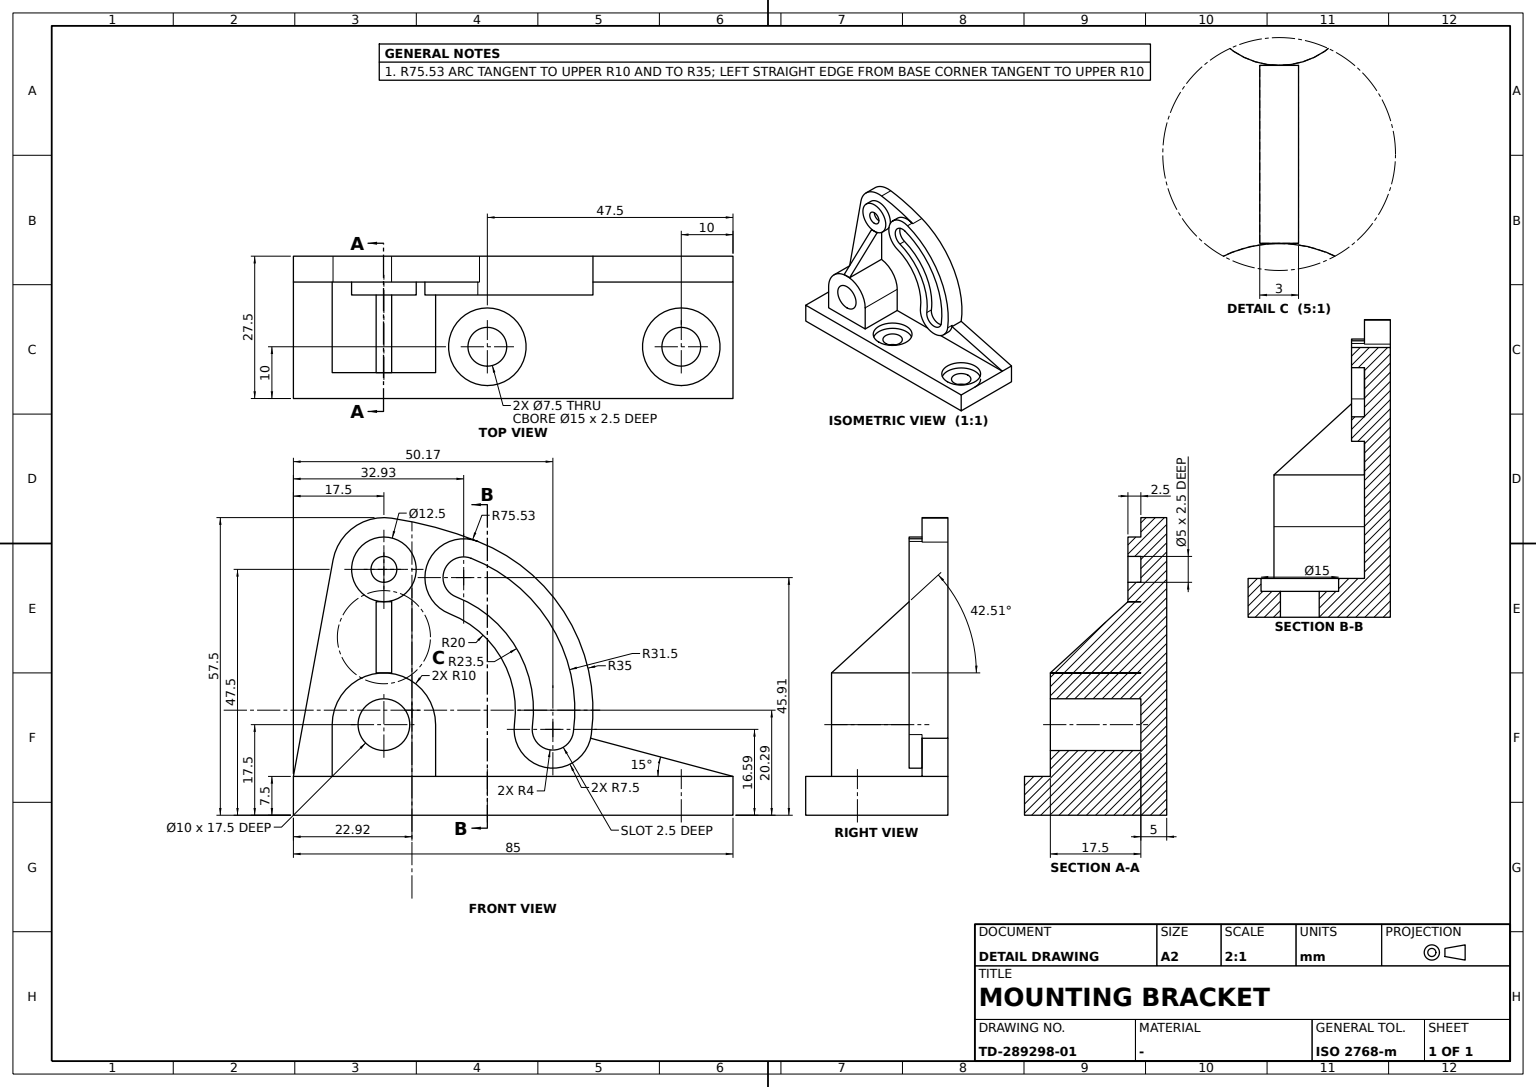
ISO-10303-21;
HEADER;
FILE_DESCRIPTION((''),'2;1');
FILE_NAME('','',(''),(''),'','','');
FILE_SCHEMA(('AUTOMOTIVE_DESIGN'));
ENDSEC;
DATA;
#1=APPLICATION_CONTEXT('');
#2=PRODUCT_CONTEXT('',#1,'mechanical');
#3=PRODUCT('','','',(#2));
#4=PRODUCT_DEFINITION_FORMATION('','',#3);
#5=PRODUCT_DEFINITION_CONTEXT('',#1,'design');
#6=PRODUCT_DEFINITION('','',#4,#5);
#7=PRODUCT_DEFINITION_SHAPE('','',#6);
#8=(LENGTH_UNIT()NAMED_UNIT(*)SI_UNIT(.MILLI.,.METRE.));
#9=(NAMED_UNIT(*)PLANE_ANGLE_UNIT()SI_UNIT($,.RADIAN.));
#10=(NAMED_UNIT(*)SI_UNIT($,.STERADIAN.)SOLID_ANGLE_UNIT());
#11=UNCERTAINTY_MEASURE_WITH_UNIT(LENGTH_MEASURE(0.005),#8,'distance_accuracy_value','');
#12=(GEOMETRIC_REPRESENTATION_CONTEXT(3)GLOBAL_UNCERTAINTY_ASSIGNED_CONTEXT((#11))GLOBAL_UNIT_ASSIGNED_CONTEXT((#8,#9,#10))REPRESENTATION_CONTEXT('',''));
#13=CARTESIAN_POINT('',(-3.75,-5.,5.));
#14=VERTEX_POINT('',#13);
#15=CARTESIAN_POINT('',(3.75,-5.,5.));
#16=DIRECTION('',(0.,0.,-1.));
#17=DIRECTION('',(-1.,0.,0.));
#18=AXIS2_PLACEMENT_3D('',#15,#16,#17);
#19=CIRCLE('',#18,7.5);
#20=EDGE_CURVE('',#14,#14,#19,.T.);
#21=ORIENTED_EDGE('',*,*,#20,.F.);
#22=EDGE_LOOP('',(#21));
#23=FACE_BOUND('',#22,.T.);
#24=CARTESIAN_POINT('',(0.,-5.,5.));
#25=VERTEX_POINT('',#24);
#26=CIRCLE('',#18,3.75);
#27=EDGE_CURVE('',#25,#25,#26,.T.);
#28=ORIENTED_EDGE('',*,*,#27,.T.);
#29=EDGE_LOOP('',(#28));
#30=FACE_BOUND('',#29,.T.);
#31=CARTESIAN_POINT('',(7.5,32.5,5.));
#32=DIRECTION('',(1.,0.,0.));
#33=AXIS2_PLACEMENT_3D('',#31,#16,#32);
#34=PLANE('',#33);
#35=ADVANCED_FACE('',(#23,#30),#34,.F.);
#36=CARTESIAN_POINT('',(13.75,42.5,0.));
#37=VERTEX_POINT('',#36);
#38=CARTESIAN_POINT('',(13.75,-42.5,0.));
#39=VERTEX_POINT('',#38);
#40=CARTESIAN_POINT('',(13.75,0.,0.));
#41=DIRECTION('',(0.,-1.,0.));
#42=VECTOR('',#41,1000.);
#43=LINE('',#40,#42);
#44=EDGE_CURVE('',#37,#39,#43,.T.);
#45=ORIENTED_EDGE('',*,*,#44,.F.);
#46=CARTESIAN_POINT('',(13.75,42.5,7.5));
#47=VERTEX_POINT('',#46);
#48=DIRECTION('',(0.,0.,1.));
#49=VECTOR('',#48,1000.);
#50=LINE('',#36,#49);
#51=EDGE_CURVE('',#37,#47,#50,.T.);
#52=ORIENTED_EDGE('',*,*,#51,.T.);
#53=CARTESIAN_POINT('',(13.75,-42.5,7.5));
#54=VERTEX_POINT('',#53);
#55=CARTESIAN_POINT('',(13.75,0.,7.5));
#56=LINE('',#55,#42);
#57=EDGE_CURVE('',#47,#54,#56,.T.);
#58=ORIENTED_EDGE('',*,*,#57,.T.);
#59=LINE('',#38,#49);
#60=EDGE_CURVE('',#39,#54,#59,.T.);
#61=ORIENTED_EDGE('',*,*,#60,.F.);
#62=EDGE_LOOP('',(#45,#52,#58,#61));
#63=FACE_BOUND('',#62,.T.);
#64=AXIS2_PLACEMENT_3D('',#36,#17,#41);
#65=PLANE('',#64);
#66=ADVANCED_FACE('',(#63),#65,.F.);
#67=CARTESIAN_POINT('',(-13.75,-34.836066,49.303279));
#68=VERTEX_POINT('',#67);
#69=CARTESIAN_POINT('',(-13.75,-42.5,7.5));
#70=VERTEX_POINT('',#69);
#71=CARTESIAN_POINT('',(-13.75,-43.830288,0.243886));
#72=DIRECTION('',(0.,-0.180327869,-0.983606557));
#73=VECTOR('',#72,1000.);
#74=LINE('',#71,#73);
#75=EDGE_CURVE('',#68,#70,#74,.T.);
#76=ORIENTED_EDGE('',*,*,#75,.T.);
#77=CARTESIAN_POINT('',(-8.75,-42.5,7.5));
#78=VERTEX_POINT('',#77);
#79=VECTOR('',#32,1000.);
#80=LINE('',#53,#79);
#81=EDGE_CURVE('',#70,#78,#80,.T.);
#82=ORIENTED_EDGE('',*,*,#81,.T.);
#83=CARTESIAN_POINT('',(-8.75,-34.836066,49.303279));
#84=VERTEX_POINT('',#83);
#85=LINE('',#83,#73);
#86=EDGE_CURVE('',#84,#78,#85,.T.);
#87=ORIENTED_EDGE('',*,*,#86,.F.);
#88=CARTESIAN_POINT('',(-11.25,-34.836066,49.303279));
#89=VECTOR('',#17,1000.);
#90=LINE('',#88,#89);
#91=EDGE_CURVE('',#68,#84,#90,.F.);
#92=ORIENTED_EDGE('',*,*,#91,.F.);
#93=EDGE_LOOP('',(#76,#82,#87,#92));
#94=FACE_BOUND('',#93,.T.);
#95=DIRECTION('',(0.,-0.983606557,0.180327869));
#96=AXIS2_PLACEMENT_3D('',#67,#95,#72);
#97=PLANE('',#96);
#98=ADVANCED_FACE('',(#94),#97,.T.);
#99=CARTESIAN_POINT('',(-13.75,-42.5,0.));
#100=VERTEX_POINT('',#99);
#101=CARTESIAN_POINT('',(0.,-42.5,0.));
#102=LINE('',#101,#89);
#103=EDGE_CURVE('',#39,#100,#102,.T.);
#104=ORIENTED_EDGE('',*,*,#103,.F.);
#105=ORIENTED_EDGE('',*,*,#60,.T.);
#106=CARTESIAN_POINT('',(0.,-42.5,7.5));
#107=LINE('',#106,#89);
#108=EDGE_CURVE('',#54,#78,#107,.T.);
#109=ORIENTED_EDGE('',*,*,#108,.T.);
#110=ORIENTED_EDGE('',*,*,#81,.F.);
#111=LINE('',#99,#49);
#112=EDGE_CURVE('',#100,#70,#111,.T.);
#113=ORIENTED_EDGE('',*,*,#112,.F.);
#114=EDGE_LOOP('',(#104,#105,#109,#110,#113));
#115=FACE_BOUND('',#114,.T.);
#116=DIRECTION('',(0.,1.,0.));
#117=AXIS2_PLACEMENT_3D('',#38,#116,#17);
#118=PLANE('',#117);
#119=ADVANCED_FACE('',(#115),#118,.F.);
#120=CARTESIAN_POINT('',(7.5,32.5,0.));
#121=VERTEX_POINT('',#120);
#122=CARTESIAN_POINT('',(3.75,32.5,0.));
#123=AXIS2_PLACEMENT_3D('',#122,#48,#32);
#124=CIRCLE('',#123,3.75);
#125=EDGE_CURVE('',#121,#121,#124,.T.);
#126=ORIENTED_EDGE('',*,*,#125,.F.);
#127=EDGE_LOOP('',(#126));
#128=FACE_BOUND('',#127,.T.);
#129=CARTESIAN_POINT('',(0.,32.5,5.));
#130=VERTEX_POINT('',#129);
#131=CARTESIAN_POINT('',(3.75,32.5,5.));
#132=AXIS2_PLACEMENT_3D('',#131,#16,#17);
#133=CIRCLE('',#132,3.75);
#134=EDGE_CURVE('',#130,#130,#133,.T.);
#135=ORIENTED_EDGE('',*,*,#134,.F.);
#136=EDGE_LOOP('',(#135));
#137=FACE_BOUND('',#136,.T.);
#138=CARTESIAN_POINT('',(3.75,32.5,7.4));
#139=AXIS2_PLACEMENT_3D('',#138,#16,#32);
#140=CYLINDRICAL_SURFACE('',#139,3.75);
#141=ADVANCED_FACE('',(#128,#137),#140,.F.);
#142=CARTESIAN_POINT('',(-8.75,-15.,17.5));
#143=VERTEX_POINT('',#142);
#144=CARTESIAN_POINT('',(-8.75,-15.,7.5));
#145=VERTEX_POINT('',#144);
#146=VECTOR('',#16,1000.);
#147=LINE('',#142,#146);
#148=EDGE_CURVE('',#143,#145,#147,.T.);
#149=ORIENTED_EDGE('',*,*,#148,.T.);
#150=CARTESIAN_POINT('',(-8.75,42.5,7.5));
#151=VERTEX_POINT('',#150);
#152=CARTESIAN_POINT('',(-8.75,0.,7.5));
#153=LINE('',#152,#42);
#154=EDGE_CURVE('',#151,#145,#153,.T.);
#155=ORIENTED_EDGE('',*,*,#154,.F.);
#156=CARTESIAN_POINT('',(-8.75,14.986884,14.871731));
#157=VERTEX_POINT('',#156);
#158=DIRECTION('',(0.,-0.965925826,0.258819045));
#159=VECTOR('',#158,1000.);
#160=LINE('',#150,#159);
#161=EDGE_CURVE('',#151,#157,#160,.T.);
#162=ORIENTED_EDGE('',*,*,#161,.T.);
#163=CARTESIAN_POINT('',(-8.75,0.24077,17.599853));
#164=VERTEX_POINT('',#163);
#165=CARTESIAN_POINT('',(-8.75,7.672397,16.589451));
#166=AXIS2_PLACEMENT_3D('',#165,#17,#48);
#167=CIRCLE('',#166,7.5);
#168=EDGE_CURVE('',#164,#157,#167,.F.);
#169=ORIENTED_EDGE('',*,*,#168,.F.);
#170=CARTESIAN_POINT('',(-8.75,-12.300381,38.923598));
#171=VERTEX_POINT('',#170);
#172=CARTESIAN_POINT('',(-8.75,-19.576903,20.29426));
#173=AXIS2_PLACEMENT_3D('',#172,#17,#48);
#174=CIRCLE('',#173,20.);
#175=EDGE_CURVE('',#164,#171,#174,.F.);
#176=ORIENTED_EDGE('',*,*,#175,.T.);
#177=CARTESIAN_POINT('',(-8.75,-6.842813,52.896043));
#178=VERTEX_POINT('',#177);
#179=CARTESIAN_POINT('',(-8.75,-9.571685,45.9096));
#180=AXIS2_PLACEMENT_3D('',#179,#17,#48);
#181=CIRCLE('',#180,7.5);
#182=EDGE_CURVE('',#178,#171,#181,.F.);
#183=ORIENTED_EDGE('',*,*,#182,.F.);
#184=CARTESIAN_POINT('',(-8.75,-23.519463,57.389793));
#185=VERTEX_POINT('',#184);
#186=CARTESIAN_POINT('',(-8.75,-34.702133,-17.308958));
#187=AXIS2_PLACEMENT_3D('',#186,#17,#48);
#188=CIRCLE('',#187,75.531156);
#189=EDGE_CURVE('',#185,#178,#188,.T.);
#190=ORIENTED_EDGE('',*,*,#189,.F.);
#191=CARTESIAN_POINT('',(-8.75,-25.,47.5));
#192=AXIS2_PLACEMENT_3D('',#191,#17,#48);
#193=CIRCLE('',#192,10.);
#194=EDGE_CURVE('',#84,#185,#193,.T.);
#195=ORIENTED_EDGE('',*,*,#194,.F.);
#196=ORIENTED_EDGE('',*,*,#86,.T.);
#197=CARTESIAN_POINT('',(-8.75,-35.,7.5));
#198=VERTEX_POINT('',#197);
#199=EDGE_CURVE('',#198,#78,#153,.T.);
#200=ORIENTED_EDGE('',*,*,#199,.F.);
#201=CARTESIAN_POINT('',(-8.75,-35.,17.5));
#202=VERTEX_POINT('',#201);
#203=LINE('',#201,#146);
#204=EDGE_CURVE('',#202,#198,#203,.T.);
#205=ORIENTED_EDGE('',*,*,#204,.F.);
#206=CARTESIAN_POINT('',(-8.75,-25.,27.5));
#207=VERTEX_POINT('',#206);
#208=CARTESIAN_POINT('',(-8.75,-25.,17.5));
#209=AXIS2_PLACEMENT_3D('',#208,#17,#48);
#210=CIRCLE('',#209,10.);
#211=EDGE_CURVE('',#202,#207,#210,.T.);
#212=ORIENTED_EDGE('',*,*,#211,.T.);
#213=CARTESIAN_POINT('',(-8.75,-26.5,27.5));
#214=VERTEX_POINT('',#213);
#215=VECTOR('',#116,1000.);
#216=LINE('',#206,#215);
#217=EDGE_CURVE('',#214,#207,#216,.T.);
#218=ORIENTED_EDGE('',*,*,#217,.F.);
#219=CARTESIAN_POINT('',(-8.75,-26.5,41.25));
#220=VERTEX_POINT('',#219);
#221=CARTESIAN_POINT('',(-8.75,-26.5,0.));
#222=LINE('',#221,#146);
#223=EDGE_CURVE('',#220,#214,#222,.T.);
#224=ORIENTED_EDGE('',*,*,#223,.F.);
#225=CARTESIAN_POINT('',(-8.75,-25.,41.25));
#226=VERTEX_POINT('',#225);
#227=LINE('',#225,#215);
#228=EDGE_CURVE('',#220,#226,#227,.T.);
#229=ORIENTED_EDGE('',*,*,#228,.T.);
#230=CIRCLE('',#192,6.25);
#231=EDGE_CURVE('',#226,#226,#230,.T.);
#232=ORIENTED_EDGE('',*,*,#231,.T.);
#233=CARTESIAN_POINT('',(-8.75,-23.5,41.25));
#234=VERTEX_POINT('',#233);
#235=EDGE_CURVE('',#226,#234,#227,.T.);
#236=ORIENTED_EDGE('',*,*,#235,.T.);
#237=CARTESIAN_POINT('',(-8.75,-23.5,27.5));
#238=VERTEX_POINT('',#237);
#239=CARTESIAN_POINT('',(-8.75,-23.5,0.));
#240=LINE('',#239,#146);
#241=EDGE_CURVE('',#234,#238,#240,.T.);
#242=ORIENTED_EDGE('',*,*,#241,.T.);
#243=EDGE_CURVE('',#207,#238,#216,.T.);
#244=ORIENTED_EDGE('',*,*,#243,.F.);
#245=EDGE_CURVE('',#207,#143,#210,.T.);
#246=ORIENTED_EDGE('',*,*,#245,.T.);
#247=EDGE_LOOP('',(#149,#155,#162,#169,#176,#183,#190,#195,#196,#200,#205,#212,#218,#224,#229,#232,#236,#242,#244,#246));
#248=FACE_BOUND('',#247,.T.);
#249=CARTESIAN_POINT('',(-8.75,0.,0.));
#250=AXIS2_PLACEMENT_3D('',#249,#17,#41);
#251=PLANE('',#250);
#252=ADVANCED_FACE('',(#248),#251,.F.);
#253=CARTESIAN_POINT('',(7.5,-5.,0.));
#254=VERTEX_POINT('',#253);
#255=CARTESIAN_POINT('',(3.75,-5.,0.));
#256=AXIS2_PLACEMENT_3D('',#255,#48,#32);
#257=CIRCLE('',#256,3.75);
#258=EDGE_CURVE('',#254,#254,#257,.T.);
#259=ORIENTED_EDGE('',*,*,#258,.F.);
#260=EDGE_LOOP('',(#259));
#261=FACE_BOUND('',#260,.T.);
#262=ORIENTED_EDGE('',*,*,#27,.F.);
#263=EDGE_LOOP('',(#262));
#264=FACE_BOUND('',#263,.T.);
#265=CARTESIAN_POINT('',(3.75,-5.,7.4));
#266=AXIS2_PLACEMENT_3D('',#265,#16,#32);
#267=CYLINDRICAL_SURFACE('',#266,3.75);
#268=ADVANCED_FACE('',(#261,#264),#267,.F.);
#269=CARTESIAN_POINT('',(-6.25,-26.5,41.25));
#270=VERTEX_POINT('',#269);
#271=CARTESIAN_POINT('',(-6.25,-23.5,41.25));
#272=VERTEX_POINT('',#271);
#273=CARTESIAN_POINT('',(-6.25,-25.,41.25));
#274=LINE('',#273,#215);
#275=EDGE_CURVE('',#270,#272,#274,.T.);
#276=ORIENTED_EDGE('',*,*,#275,.F.);
#277=CARTESIAN_POINT('',(8.75,-26.5,27.5));
#278=VERTEX_POINT('',#277);
#279=CARTESIAN_POINT('',(17.693396,-26.5,19.301887));
#280=DIRECTION('',(0.73715414,0.,-0.675724629));
#281=VECTOR('',#280,1000.);
#282=LINE('',#279,#281);
#283=EDGE_CURVE('',#270,#278,#282,.T.);
#284=ORIENTED_EDGE('',*,*,#283,.T.);
#285=CARTESIAN_POINT('',(8.75,-23.5,27.5));
#286=VERTEX_POINT('',#285);
#287=CARTESIAN_POINT('',(8.75,-25.,27.5));
#288=LINE('',#287,#215);
#289=EDGE_CURVE('',#278,#286,#288,.T.);
#290=ORIENTED_EDGE('',*,*,#289,.T.);
#291=CARTESIAN_POINT('',(17.693396,-23.5,19.301887));
#292=LINE('',#291,#281);
#293=EDGE_CURVE('',#272,#286,#292,.T.);
#294=ORIENTED_EDGE('',*,*,#293,.F.);
#295=EDGE_LOOP('',(#276,#284,#290,#294));
#296=FACE_BOUND('',#295,.T.);
#297=DIRECTION('',(0.675724629,0.,0.73715414));
#298=AXIS2_PLACEMENT_3D('',#273,#297,#280);
#299=PLANE('',#298);
#300=ADVANCED_FACE('',(#296),#299,.T.);
#301=ORIENTED_EDGE('',*,*,#161,.F.);
#302=CARTESIAN_POINT('',(-13.75,42.5,7.5));
#303=VERTEX_POINT('',#302);
#304=LINE('',#302,#79);
#305=EDGE_CURVE('',#303,#151,#304,.T.);
#306=ORIENTED_EDGE('',*,*,#305,.F.);
#307=CARTESIAN_POINT('',(-13.75,15.,14.868603));
#308=VERTEX_POINT('',#307);
#309=CARTESIAN_POINT('',(-13.75,-34.93108,28.247595));
#310=LINE('',#309,#159);
#311=EDGE_CURVE('',#303,#308,#310,.T.);
#312=ORIENTED_EDGE('',*,*,#311,.T.);
#313=LINE('',#307,#79);
#314=EDGE_CURVE('',#308,#157,#313,.T.);
#315=ORIENTED_EDGE('',*,*,#314,.T.);
#316=EDGE_LOOP('',(#301,#306,#312,#315));
#317=FACE_BOUND('',#316,.T.);
#318=DIRECTION('',(0.,0.258819045,0.965925826));
#319=AXIS2_PLACEMENT_3D('',#302,#318,#158);
#320=PLANE('',#319);
#321=ADVANCED_FACE('',(#317),#320,.T.);
#322=CARTESIAN_POINT('',(8.75,-15.,7.5));
#323=VERTEX_POINT('',#322);
#324=CARTESIAN_POINT('',(0.,-15.,7.5));
#325=LINE('',#324,#79);
#326=EDGE_CURVE('',#145,#323,#325,.T.);
#327=ORIENTED_EDGE('',*,*,#326,.F.);
#328=ORIENTED_EDGE('',*,*,#148,.F.);
#329=CARTESIAN_POINT('',(8.75,-15.,17.5));
#330=VERTEX_POINT('',#329);
#331=CARTESIAN_POINT('',(0.,-15.,17.5));
#332=LINE('',#331,#79);
#333=EDGE_CURVE('',#143,#330,#332,.T.);
#334=ORIENTED_EDGE('',*,*,#333,.T.);
#335=CARTESIAN_POINT('',(8.75,-15.,0.));
#336=LINE('',#335,#146);
#337=EDGE_CURVE('',#330,#323,#336,.T.);
#338=ORIENTED_EDGE('',*,*,#337,.T.);
#339=EDGE_LOOP('',(#327,#328,#334,#338));
#340=FACE_BOUND('',#339,.T.);
#341=AXIS2_PLACEMENT_3D('',#142,#41,#16);
#342=PLANE('',#341);
#343=ADVANCED_FACE('',(#340),#342,.F.);
#344=CARTESIAN_POINT('',(-8.75,-25.,50.));
#345=VERTEX_POINT('',#344);
#346=CIRCLE('',#192,2.5);
#347=EDGE_CURVE('',#345,#345,#346,.T.);
#348=ORIENTED_EDGE('',*,*,#347,.F.);
#349=EDGE_LOOP('',(#348));
#350=FACE_BOUND('',#349,.T.);
#351=ADVANCED_FACE('',(#350),#251,.F.);
#352=CARTESIAN_POINT('',(-6.25,-25.,45.));
#353=VERTEX_POINT('',#352);
#354=CARTESIAN_POINT('',(-6.25,-25.,47.5));
#355=AXIS2_PLACEMENT_3D('',#354,#32,#16);
#356=CIRCLE('',#355,2.5);
#357=EDGE_CURVE('',#353,#353,#356,.T.);
#358=ORIENTED_EDGE('',*,*,#357,.F.);
#359=EDGE_LOOP('',(#358));
#360=FACE_BOUND('',#359,.T.);
#361=VERTEX_POINT('',#273);
#362=CIRCLE('',#355,6.25);
#363=EDGE_CURVE('',#361,#361,#362,.T.);
#364=ORIENTED_EDGE('',*,*,#363,.T.);
#365=EDGE_LOOP('',(#364));
#366=FACE_BOUND('',#365,.T.);
#367=CARTESIAN_POINT('',(-6.25,0.,0.));
#368=AXIS2_PLACEMENT_3D('',#367,#32,#116);
#369=PLANE('',#368);
#370=ADVANCED_FACE('',(#360,#366),#369,.T.);
#371=ORIENTED_EDGE('',*,*,#235,.F.);
#372=ORIENTED_EDGE('',*,*,#228,.F.);
#373=CARTESIAN_POINT('',(0.,-26.5,41.25));
#374=LINE('',#373,#89);
#375=EDGE_CURVE('',#270,#220,#374,.T.);
#376=ORIENTED_EDGE('',*,*,#375,.F.);
#377=ORIENTED_EDGE('',*,*,#275,.T.);
#378=CARTESIAN_POINT('',(0.,-23.5,41.25));
#379=LINE('',#378,#89);
#380=EDGE_CURVE('',#272,#234,#379,.T.);
#381=ORIENTED_EDGE('',*,*,#380,.T.);
#382=EDGE_LOOP('',(#371,#372,#376,#377,#381));
#383=FACE_BOUND('',#382,.T.);
#384=AXIS2_PLACEMENT_3D('',#273,#16,#17);
#385=PLANE('',#384);
#386=ADVANCED_FACE('',(#383),#385,.F.);
#387=ORIENTED_EDGE('',*,*,#333,.F.);
#388=ORIENTED_EDGE('',*,*,#245,.F.);
#389=ORIENTED_EDGE('',*,*,#211,.F.);
#390=CARTESIAN_POINT('',(8.75,-35.,17.5));
#391=VERTEX_POINT('',#390);
#392=CARTESIAN_POINT('',(0.,-35.,17.5));
#393=LINE('',#392,#79);
#394=EDGE_CURVE('',#202,#391,#393,.T.);
#395=ORIENTED_EDGE('',*,*,#394,.T.);
#396=CARTESIAN_POINT('',(8.75,-25.,17.5));
#397=AXIS2_PLACEMENT_3D('',#396,#32,#16);
#398=CIRCLE('',#397,10.);
#399=EDGE_CURVE('',#330,#391,#398,.T.);
#400=ORIENTED_EDGE('',*,*,#399,.F.);
#401=EDGE_LOOP('',(#387,#388,#389,#395,#400));
#402=FACE_BOUND('',#401,.T.);
#403=CARTESIAN_POINT('',(0.,-25.,17.5));
#404=AXIS2_PLACEMENT_3D('',#403,#32,#116);
#405=CYLINDRICAL_SURFACE('',#404,10.);
#406=ADVANCED_FACE('',(#402),#405,.T.);
#407=CARTESIAN_POINT('',(-8.75,-8.11638,49.635467));
#408=VERTEX_POINT('',#407);
#409=CARTESIAN_POINT('',(-6.25,-8.11638,49.635467));
#410=VERTEX_POINT('',#409);
#411=CARTESIAN_POINT('',(-7.5,-8.11638,49.635467));
#412=LINE('',#411,#79);
#413=EDGE_CURVE('',#408,#410,#412,.T.);
#414=ORIENTED_EDGE('',*,*,#413,.F.);
#415=CARTESIAN_POINT('',(-8.75,11.635932,16.050569));
#416=VERTEX_POINT('',#415);
#417=CIRCLE('',#173,31.5);
#418=EDGE_CURVE('',#416,#408,#417,.F.);
#419=ORIENTED_EDGE('',*,*,#418,.F.);
#420=CARTESIAN_POINT('',(-6.25,11.635932,16.050569));
#421=VERTEX_POINT('',#420);
#422=CARTESIAN_POINT('',(-7.5,11.635932,16.050569));
#423=LINE('',#422,#79);
#424=EDGE_CURVE('',#416,#421,#423,.T.);
#425=ORIENTED_EDGE('',*,*,#424,.T.);
#426=CARTESIAN_POINT('',(-6.25,-19.576903,20.29426));
#427=AXIS2_PLACEMENT_3D('',#426,#32,#16);
#428=CIRCLE('',#427,31.5);
#429=EDGE_CURVE('',#421,#410,#428,.T.);
#430=ORIENTED_EDGE('',*,*,#429,.T.);
#431=EDGE_LOOP('',(#414,#419,#425,#430));
#432=FACE_BOUND('',#431,.T.);
#433=CARTESIAN_POINT('',(-7.5,-19.576903,20.29426));
#434=AXIS2_PLACEMENT_3D('',#433,#32,#116);
#435=CYLINDRICAL_SURFACE('',#434,31.5);
#436=ADVANCED_FACE('',(#432),#435,.F.);
#437=CARTESIAN_POINT('',(-8.75,-25.,22.5));
#438=VERTEX_POINT('',#437);
#439=CIRCLE('',#209,5.);
#440=EDGE_CURVE('',#438,#438,#439,.T.);
#441=ORIENTED_EDGE('',*,*,#440,.F.);
#442=EDGE_LOOP('',(#441));
#443=FACE_BOUND('',#442,.T.);
#444=ADVANCED_FACE('',(#443),#251,.F.);
#445=ORIENTED_EDGE('',*,*,#258,.T.);
#446=EDGE_LOOP('',(#445));
#447=FACE_BOUND('',#446,.T.);
#448=CARTESIAN_POINT('',(-13.75,42.5,0.));
#449=VERTEX_POINT('',#448);
#450=CARTESIAN_POINT('',(0.,42.5,0.));
#451=LINE('',#450,#79);
#452=EDGE_CURVE('',#449,#37,#451,.T.);
#453=ORIENTED_EDGE('',*,*,#452,.T.);
#454=ORIENTED_EDGE('',*,*,#44,.T.);
#455=ORIENTED_EDGE('',*,*,#103,.T.);
#456=CARTESIAN_POINT('',(-13.75,0.,0.));
#457=LINE('',#456,#215);
#458=EDGE_CURVE('',#100,#449,#457,.T.);
#459=ORIENTED_EDGE('',*,*,#458,.T.);
#460=EDGE_LOOP('',(#453,#454,#455,#459));
#461=FACE_BOUND('',#460,.T.);
#462=ORIENTED_EDGE('',*,*,#125,.T.);
#463=EDGE_LOOP('',(#462));
#464=FACE_BOUND('',#463,.T.);
#465=CARTESIAN_POINT('',(0.,0.,0.));
#466=AXIS2_PLACEMENT_3D('',#465,#48,#32);
#467=PLANE('',#466);
#468=ADVANCED_FACE('',(#447,#461,#464),#467,.F.);
#469=ORIENTED_EDGE('',*,*,#134,.T.);
#470=EDGE_LOOP('',(#469));
#471=FACE_BOUND('',#470,.T.);
#472=CARTESIAN_POINT('',(-3.75,32.5,5.));
#473=VERTEX_POINT('',#472);
#474=CIRCLE('',#132,7.5);
#475=EDGE_CURVE('',#473,#473,#474,.T.);
#476=ORIENTED_EDGE('',*,*,#475,.F.);
#477=EDGE_LOOP('',(#476));
#478=FACE_BOUND('',#477,.T.);
#479=ADVANCED_FACE('',(#471,#478),#34,.F.);
#480=ORIENTED_EDGE('',*,*,#293,.T.);
#481=CARTESIAN_POINT('',(0.,-23.5,27.5));
#482=LINE('',#481,#89);
#483=EDGE_CURVE('',#286,#238,#482,.T.);
#484=ORIENTED_EDGE('',*,*,#483,.T.);
#485=ORIENTED_EDGE('',*,*,#241,.F.);
#486=ORIENTED_EDGE('',*,*,#380,.F.);
#487=EDGE_LOOP('',(#480,#484,#485,#486));
#488=FACE_BOUND('',#487,.T.);
#489=CARTESIAN_POINT('',(0.,-23.5,0.));
#490=AXIS2_PLACEMENT_3D('',#489,#116,#17);
#491=PLANE('',#490);
#492=ADVANCED_FACE('',(#488),#491,.T.);
#493=CARTESIAN_POINT('',(8.75,-35.,7.5));
#494=VERTEX_POINT('',#493);
#495=CARTESIAN_POINT('',(8.75,0.,7.5));
#496=LINE('',#495,#215);
#497=EDGE_CURVE('',#494,#323,#496,.T.);
#498=ORIENTED_EDGE('',*,*,#497,.T.);
#499=ORIENTED_EDGE('',*,*,#337,.F.);
#500=ORIENTED_EDGE('',*,*,#399,.T.);
#501=CARTESIAN_POINT('',(8.75,-35.,0.));
#502=LINE('',#501,#146);
#503=EDGE_CURVE('',#391,#494,#502,.T.);
#504=ORIENTED_EDGE('',*,*,#503,.T.);
#505=EDGE_LOOP('',(#498,#499,#500,#504));
#506=FACE_BOUND('',#505,.T.);
#507=CARTESIAN_POINT('',(8.75,-25.,12.5));
#508=VERTEX_POINT('',#507);
#509=CIRCLE('',#397,5.);
#510=EDGE_CURVE('',#508,#508,#509,.T.);
#511=ORIENTED_EDGE('',*,*,#510,.F.);
#512=EDGE_LOOP('',(#511));
#513=FACE_BOUND('',#512,.T.);
#514=CARTESIAN_POINT('',(8.75,0.,0.));
#515=AXIS2_PLACEMENT_3D('',#514,#32,#116);
#516=PLANE('',#515);
#517=ADVANCED_FACE('',(#506,#513),#516,.T.);
#518=ORIENTED_EDGE('',*,*,#283,.F.);
#519=ORIENTED_EDGE('',*,*,#375,.T.);
#520=ORIENTED_EDGE('',*,*,#223,.T.);
#521=CARTESIAN_POINT('',(0.,-26.5,27.5));
#522=LINE('',#521,#89);
#523=EDGE_CURVE('',#278,#214,#522,.T.);
#524=ORIENTED_EDGE('',*,*,#523,.F.);
#525=EDGE_LOOP('',(#518,#519,#520,#524));
#526=FACE_BOUND('',#525,.T.);
#527=CARTESIAN_POINT('',(0.,-26.5,0.));
#528=AXIS2_PLACEMENT_3D('',#527,#116,#17);
#529=PLANE('',#528);
#530=ADVANCED_FACE('',(#526),#529,.F.);
#531=CARTESIAN_POINT('',(11.25,-5.,7.5));
#532=VERTEX_POINT('',#531);
#533=CARTESIAN_POINT('',(3.75,-5.,7.5));
#534=AXIS2_PLACEMENT_3D('',#533,#48,#32);
#535=CIRCLE('',#534,7.5);
#536=EDGE_CURVE('',#532,#532,#535,.T.);
#537=ORIENTED_EDGE('',*,*,#536,.F.);
#538=EDGE_LOOP('',(#537));
#539=FACE_BOUND('',#538,.T.);
#540=ORIENTED_EDGE('',*,*,#199,.T.);
#541=ORIENTED_EDGE('',*,*,#108,.F.);
#542=ORIENTED_EDGE('',*,*,#57,.F.);
#543=CARTESIAN_POINT('',(0.,42.5,7.5));
#544=LINE('',#543,#79);
#545=EDGE_CURVE('',#151,#47,#544,.T.);
#546=ORIENTED_EDGE('',*,*,#545,.F.);
#547=ORIENTED_EDGE('',*,*,#154,.T.);
#548=ORIENTED_EDGE('',*,*,#326,.T.);
#549=ORIENTED_EDGE('',*,*,#497,.F.);
#550=CARTESIAN_POINT('',(0.,-35.,7.5));
#551=LINE('',#550,#79);
#552=EDGE_CURVE('',#198,#494,#551,.T.);
#553=ORIENTED_EDGE('',*,*,#552,.F.);
#554=EDGE_LOOP('',(#540,#541,#542,#546,#547,#548,#549,#553));
#555=FACE_BOUND('',#554,.T.);
#556=CARTESIAN_POINT('',(11.25,32.5,7.5));
#557=VERTEX_POINT('',#556);
#558=CARTESIAN_POINT('',(3.75,32.5,7.5));
#559=AXIS2_PLACEMENT_3D('',#558,#48,#32);
#560=CIRCLE('',#559,7.5);
#561=EDGE_CURVE('',#557,#557,#560,.T.);
#562=ORIENTED_EDGE('',*,*,#561,.F.);
#563=EDGE_LOOP('',(#562));
#564=FACE_BOUND('',#563,.T.);
#565=CARTESIAN_POINT('',(0.,0.,7.5));
#566=AXIS2_PLACEMENT_3D('',#565,#48,#32);
#567=PLANE('',#566);
#568=ADVANCED_FACE('',(#539,#555,#564),#567,.T.);
#569=CARTESIAN_POINT('',(-13.75,-23.519463,57.389793));
#570=VERTEX_POINT('',#569);
#571=CARTESIAN_POINT('',(-13.75,-25.,47.5));
#572=AXIS2_PLACEMENT_3D('',#571,#32,#16);
#573=CIRCLE('',#572,10.);
#574=EDGE_CURVE('',#68,#570,#573,.F.);
#575=ORIENTED_EDGE('',*,*,#574,.F.);
#576=ORIENTED_EDGE('',*,*,#91,.T.);
#577=ORIENTED_EDGE('',*,*,#194,.T.);
#578=CARTESIAN_POINT('',(-11.25,-23.519463,57.389793));
#579=LINE('',#578,#89);
#580=EDGE_CURVE('',#570,#185,#579,.F.);
#581=ORIENTED_EDGE('',*,*,#580,.F.);
#582=EDGE_LOOP('',(#575,#576,#577,#581));
#583=FACE_BOUND('',#582,.T.);
#584=CARTESIAN_POINT('',(-11.25,-25.,47.5));
#585=AXIS2_PLACEMENT_3D('',#584,#17,#41);
#586=CYLINDRICAL_SURFACE('',#585,10.);
#587=ADVANCED_FACE('',(#583),#586,.T.);
#588=CARTESIAN_POINT('',(-6.25,0.24077,17.599853));
#589=VERTEX_POINT('',#588);
#590=CARTESIAN_POINT('',(-7.5,0.24077,17.599853));
#591=LINE('',#590,#79);
#592=EDGE_CURVE('',#164,#589,#591,.T.);
#593=ORIENTED_EDGE('',*,*,#592,.F.);
#594=ORIENTED_EDGE('',*,*,#168,.T.);
#595=CARTESIAN_POINT('',(-8.75,15.104025,15.579048));
#596=VERTEX_POINT('',#595);
#597=CARTESIAN_POINT('',(-8.75,14.973768,14.874811));
#598=CARTESIAN_POINT('',(-8.75,15.028366,15.107305));
#599=CARTESIAN_POINT('',(-8.75,15.071851,15.342407));
#600=B_SPLINE_CURVE_WITH_KNOTS('',3,(#597,#598,#599,#595),.UNSPECIFIED.,.F.,.F.,(4,4),(45.393951603,46.11040549),.UNSPECIFIED.);
#601=EDGE_CURVE('',#157,#596,#600,.T.);
#602=ORIENTED_EDGE('',*,*,#601,.T.);
#603=CARTESIAN_POINT('',(-6.25,15.104025,15.579048));
#604=VERTEX_POINT('',#603);
#605=CARTESIAN_POINT('',(-7.569312,15.104025,15.579048));
#606=LINE('',#605,#79);
#607=EDGE_CURVE('',#596,#604,#606,.T.);
#608=ORIENTED_EDGE('',*,*,#607,.T.);
#609=CARTESIAN_POINT('',(-6.25,7.672397,16.589451));
#610=AXIS2_PLACEMENT_3D('',#609,#32,#16);
#611=CIRCLE('',#610,7.5);
#612=EDGE_CURVE('',#589,#604,#611,.T.);
#613=ORIENTED_EDGE('',*,*,#612,.F.);
#614=EDGE_LOOP('',(#593,#594,#602,#608,#613));
#615=FACE_BOUND('',#614,.T.);
#616=CARTESIAN_POINT('',(-7.5,7.672397,16.589451));
#617=AXIS2_PLACEMENT_3D('',#616,#32,#116);
#618=CYLINDRICAL_SURFACE('',#617,7.5);
#619=ADVANCED_FACE('',(#615),#618,.T.);
#620=ORIENTED_EDGE('',*,*,#523,.T.);
#621=ORIENTED_EDGE('',*,*,#217,.T.);
#622=ORIENTED_EDGE('',*,*,#243,.T.);
#623=ORIENTED_EDGE('',*,*,#483,.F.);
#624=ORIENTED_EDGE('',*,*,#289,.F.);
#625=EDGE_LOOP('',(#620,#621,#622,#623,#624));
#626=FACE_BOUND('',#625,.T.);
#627=AXIS2_PLACEMENT_3D('',#287,#16,#17);
#628=PLANE('',#627);
#629=ADVANCED_FACE('',(#626),#628,.T.);
#630=CARTESIAN_POINT('',(-6.25,-12.300381,38.923598));
#631=VERTEX_POINT('',#630);
#632=CIRCLE('',#427,20.);
#633=EDGE_CURVE('',#589,#631,#632,.T.);
#634=ORIENTED_EDGE('',*,*,#633,.T.);
#635=CARTESIAN_POINT('',(-7.5,-12.300381,38.923598));
#636=LINE('',#635,#79);
#637=EDGE_CURVE('',#171,#631,#636,.T.);
#638=ORIENTED_EDGE('',*,*,#637,.F.);
#639=ORIENTED_EDGE('',*,*,#175,.F.);
#640=ORIENTED_EDGE('',*,*,#592,.T.);
#641=EDGE_LOOP('',(#634,#638,#639,#640));
#642=FACE_BOUND('',#641,.T.);
#643=CYLINDRICAL_SURFACE('',#434,20.);
#644=ADVANCED_FACE('',(#642),#643,.F.);
#645=CARTESIAN_POINT('',(-6.25,-6.842989,52.895601));
#646=VERTEX_POINT('',#645);
#647=CARTESIAN_POINT('',(-7.5,-6.842989,52.895601));
#648=LINE('',#647,#79);
#649=EDGE_CURVE('',#178,#646,#648,.T.);
#650=ORIENTED_EDGE('',*,*,#649,.F.);
#651=ORIENTED_EDGE('',*,*,#182,.T.);
#652=ORIENTED_EDGE('',*,*,#637,.T.);
#653=CARTESIAN_POINT('',(-6.25,-9.571685,45.9096));
#654=AXIS2_PLACEMENT_3D('',#653,#32,#16);
#655=CIRCLE('',#654,7.5);
#656=EDGE_CURVE('',#646,#631,#655,.T.);
#657=ORIENTED_EDGE('',*,*,#656,.F.);
#658=EDGE_LOOP('',(#650,#651,#652,#657));
#659=FACE_BOUND('',#658,.T.);
#660=CARTESIAN_POINT('',(-7.5,-9.571685,45.9096));
#661=AXIS2_PLACEMENT_3D('',#660,#32,#116);
#662=CYLINDRICAL_SURFACE('',#661,7.5);
#663=ADVANCED_FACE('',(#659),#662,.T.);
#664=ORIENTED_EDGE('',*,*,#314,.F.);
#665=CARTESIAN_POINT('',(-13.75,-6.515765,52.765889));
#666=VERTEX_POINT('',#665);
#667=CARTESIAN_POINT('',(-13.75,-19.576903,20.29426));
#668=AXIS2_PLACEMENT_3D('',#667,#32,#16);
#669=CIRCLE('',#668,35.);
#670=EDGE_CURVE('',#666,#308,#669,.F.);
#671=ORIENTED_EDGE('',*,*,#670,.F.);
#672=CARTESIAN_POINT('',(-8.75,-6.515765,52.765889));
#673=VERTEX_POINT('',#672);
#674=CARTESIAN_POINT('',(-11.25,-6.515765,52.765889));
#675=LINE('',#674,#89);
#676=EDGE_CURVE('',#666,#673,#675,.F.);
#677=ORIENTED_EDGE('',*,*,#676,.T.);
#678=CARTESIAN_POINT('',(-8.75,-6.842638,52.896484));
#679=CARTESIAN_POINT('',(-8.75,-6.733579,52.853206));
#680=CARTESIAN_POINT('',(-8.75,-6.624621,52.809674));
#681=B_SPLINE_CURVE_WITH_KNOTS('',3,(#678,#679,#680,#672),.UNSPECIFIED.,.F.,.F.,(4,4),(147.177393411,147.529390033),.UNSPECIFIED.);
#682=EDGE_CURVE('',#673,#178,#681,.F.);
#683=ORIENTED_EDGE('',*,*,#682,.T.);
#684=ORIENTED_EDGE('',*,*,#649,.T.);
#685=CIRCLE('',#427,35.);
#686=EDGE_CURVE('',#604,#646,#685,.T.);
#687=ORIENTED_EDGE('',*,*,#686,.F.);
#688=ORIENTED_EDGE('',*,*,#607,.F.);
#689=ORIENTED_EDGE('',*,*,#601,.F.);
#690=EDGE_LOOP('',(#664,#671,#677,#683,#684,#687,#688,#689));
#691=FACE_BOUND('',#690,.T.);
#692=CYLINDRICAL_SURFACE('',#434,35.);
#693=ADVANCED_FACE('',(#691),#692,.T.);
#694=LINE('',#448,#49);
#695=EDGE_CURVE('',#449,#303,#694,.T.);
#696=ORIENTED_EDGE('',*,*,#695,.F.);
#697=ORIENTED_EDGE('',*,*,#458,.F.);
#698=ORIENTED_EDGE('',*,*,#112,.T.);
#699=ORIENTED_EDGE('',*,*,#75,.F.);
#700=ORIENTED_EDGE('',*,*,#574,.T.);
#701=CARTESIAN_POINT('',(-13.75,-34.702133,-17.308958));
#702=AXIS2_PLACEMENT_3D('',#701,#32,#16);
#703=CIRCLE('',#702,75.531156);
#704=EDGE_CURVE('',#570,#666,#703,.F.);
#705=ORIENTED_EDGE('',*,*,#704,.T.);
#706=ORIENTED_EDGE('',*,*,#670,.T.);
#707=ORIENTED_EDGE('',*,*,#311,.F.);
#708=EDGE_LOOP('',(#696,#697,#698,#699,#700,#705,#706,#707));
#709=FACE_BOUND('',#708,.T.);
#710=AXIS2_PLACEMENT_3D('',#99,#32,#116);
#711=PLANE('',#710);
#712=ADVANCED_FACE('',(#709),#711,.F.);
#713=ORIENTED_EDGE('',*,*,#552,.T.);
#714=ORIENTED_EDGE('',*,*,#503,.F.);
#715=ORIENTED_EDGE('',*,*,#394,.F.);
#716=ORIENTED_EDGE('',*,*,#204,.T.);
#717=EDGE_LOOP('',(#713,#714,#715,#716));
#718=FACE_BOUND('',#717,.T.);
#719=AXIS2_PLACEMENT_3D('',#201,#41,#16);
#720=PLANE('',#719);
#721=ADVANCED_FACE('',(#718),#720,.T.);
#722=ORIENTED_EDGE('',*,*,#475,.T.);
#723=EDGE_LOOP('',(#722));
#724=FACE_BOUND('',#723,.T.);
#725=ORIENTED_EDGE('',*,*,#561,.T.);
#726=EDGE_LOOP('',(#725));
#727=FACE_BOUND('',#726,.T.);
#728=CYLINDRICAL_SURFACE('',#139,7.5);
#729=ADVANCED_FACE('',(#724,#727),#728,.F.);
#730=ORIENTED_EDGE('',*,*,#418,.T.);
#731=CARTESIAN_POINT('',(-8.75,-11.026989,42.183732));
#732=VERTEX_POINT('',#731);
#733=CIRCLE('',#180,4.);
#734=EDGE_CURVE('',#408,#732,#733,.F.);
#735=ORIENTED_EDGE('',*,*,#734,.T.);
#736=CARTESIAN_POINT('',(-8.75,3.708863,17.128332));
#737=VERTEX_POINT('',#736);
#738=CIRCLE('',#173,23.5);
#739=EDGE_CURVE('',#737,#732,#738,.F.);
#740=ORIENTED_EDGE('',*,*,#739,.F.);
#741=CIRCLE('',#166,4.);
#742=EDGE_CURVE('',#737,#416,#741,.F.);
#743=ORIENTED_EDGE('',*,*,#742,.T.);
#744=EDGE_LOOP('',(#730,#735,#740,#743));
#745=FACE_BOUND('',#744,.T.);
#746=ADVANCED_FACE('',(#745),#251,.F.);
#747=ORIENTED_EDGE('',*,*,#452,.F.);
#748=ORIENTED_EDGE('',*,*,#695,.T.);
#749=ORIENTED_EDGE('',*,*,#305,.T.);
#750=ORIENTED_EDGE('',*,*,#545,.T.);
#751=ORIENTED_EDGE('',*,*,#51,.F.);
#752=EDGE_LOOP('',(#747,#748,#749,#750,#751));
#753=FACE_BOUND('',#752,.T.);
#754=AXIS2_PLACEMENT_3D('',#448,#41,#32);
#755=PLANE('',#754);
#756=ADVANCED_FACE('',(#753),#755,.F.);
#757=ORIENTED_EDGE('',*,*,#363,.F.);
#758=EDGE_LOOP('',(#757));
#759=FACE_BOUND('',#758,.T.);
#760=ORIENTED_EDGE('',*,*,#231,.F.);
#761=EDGE_LOOP('',(#760));
#762=FACE_BOUND('',#761,.T.);
#763=CARTESIAN_POINT('',(-7.5,-25.,47.5));
#764=AXIS2_PLACEMENT_3D('',#763,#32,#116);
#765=CYLINDRICAL_SURFACE('',#764,6.25);
#766=ADVANCED_FACE('',(#759,#762),#765,.T.);
#767=ORIENTED_EDGE('',*,*,#357,.T.);
#768=EDGE_LOOP('',(#767));
#769=FACE_BOUND('',#768,.T.);
#770=ORIENTED_EDGE('',*,*,#347,.T.);
#771=EDGE_LOOP('',(#770));
#772=FACE_BOUND('',#771,.T.);
#773=CYLINDRICAL_SURFACE('',#764,2.5);
#774=ADVANCED_FACE('',(#769,#772),#773,.F.);
#775=ORIENTED_EDGE('',*,*,#189,.T.);
#776=ORIENTED_EDGE('',*,*,#682,.F.);
#777=ORIENTED_EDGE('',*,*,#676,.F.);
#778=ORIENTED_EDGE('',*,*,#704,.F.);
#779=ORIENTED_EDGE('',*,*,#580,.T.);
#780=EDGE_LOOP('',(#775,#776,#777,#778,#779));
#781=FACE_BOUND('',#780,.T.);
#782=CARTESIAN_POINT('',(-11.25,-34.702133,-17.308958));
#783=AXIS2_PLACEMENT_3D('',#782,#17,#41);
#784=CYLINDRICAL_SURFACE('',#783,75.531156);
#785=ADVANCED_FACE('',(#781),#784,.T.);
#786=ORIENTED_EDGE('',*,*,#424,.F.);
#787=ORIENTED_EDGE('',*,*,#742,.F.);
#788=CARTESIAN_POINT('',(-6.25,3.708863,17.128332));
#789=VERTEX_POINT('',#788);
#790=CARTESIAN_POINT('',(-7.5,3.708863,17.128332));
#791=LINE('',#790,#79);
#792=EDGE_CURVE('',#737,#789,#791,.T.);
#793=ORIENTED_EDGE('',*,*,#792,.T.);
#794=CIRCLE('',#610,4.);
#795=EDGE_CURVE('',#789,#421,#794,.T.);
#796=ORIENTED_EDGE('',*,*,#795,.T.);
#797=EDGE_LOOP('',(#786,#787,#793,#796));
#798=FACE_BOUND('',#797,.T.);
#799=CYLINDRICAL_SURFACE('',#617,4.);
#800=ADVANCED_FACE('',(#798),#799,.F.);
#801=CARTESIAN_POINT('',(-6.25,-11.026989,42.183732));
#802=VERTEX_POINT('',#801);
#803=CIRCLE('',#654,4.);
#804=EDGE_CURVE('',#410,#802,#803,.T.);
#805=ORIENTED_EDGE('',*,*,#804,.T.);
#806=CARTESIAN_POINT('',(-7.5,-11.026989,42.183732));
#807=LINE('',#806,#79);
#808=EDGE_CURVE('',#732,#802,#807,.T.);
#809=ORIENTED_EDGE('',*,*,#808,.F.);
#810=ORIENTED_EDGE('',*,*,#734,.F.);
#811=ORIENTED_EDGE('',*,*,#413,.T.);
#812=EDGE_LOOP('',(#805,#809,#810,#811));
#813=FACE_BOUND('',#812,.T.);
#814=CYLINDRICAL_SURFACE('',#661,4.);
#815=ADVANCED_FACE('',(#813),#814,.F.);
#816=ORIENTED_EDGE('',*,*,#510,.T.);
#817=EDGE_LOOP('',(#816));
#818=FACE_BOUND('',#817,.T.);
#819=ORIENTED_EDGE('',*,*,#440,.T.);
#820=EDGE_LOOP('',(#819));
#821=FACE_BOUND('',#820,.T.);
#822=CYLINDRICAL_SURFACE('',#404,5.);
#823=ADVANCED_FACE('',(#818,#821),#822,.F.);
#824=ORIENTED_EDGE('',*,*,#686,.T.);
#825=ORIENTED_EDGE('',*,*,#656,.T.);
#826=ORIENTED_EDGE('',*,*,#633,.F.);
#827=ORIENTED_EDGE('',*,*,#612,.T.);
#828=EDGE_LOOP('',(#824,#825,#826,#827));
#829=FACE_BOUND('',#828,.T.);
#830=CIRCLE('',#427,23.5);
#831=EDGE_CURVE('',#789,#802,#830,.T.);
#832=ORIENTED_EDGE('',*,*,#831,.T.);
#833=ORIENTED_EDGE('',*,*,#804,.F.);
#834=ORIENTED_EDGE('',*,*,#429,.F.);
#835=ORIENTED_EDGE('',*,*,#795,.F.);
#836=EDGE_LOOP('',(#832,#833,#834,#835));
#837=FACE_BOUND('',#836,.T.);
#838=ADVANCED_FACE('',(#829,#837),#369,.T.);
#839=ORIENTED_EDGE('',*,*,#536,.T.);
#840=EDGE_LOOP('',(#839));
#841=FACE_BOUND('',#840,.T.);
#842=ORIENTED_EDGE('',*,*,#20,.T.);
#843=EDGE_LOOP('',(#842));
#844=FACE_BOUND('',#843,.T.);
#845=CYLINDRICAL_SURFACE('',#266,7.5);
#846=ADVANCED_FACE('',(#841,#844),#845,.F.);
#847=ORIENTED_EDGE('',*,*,#792,.F.);
#848=ORIENTED_EDGE('',*,*,#739,.T.);
#849=ORIENTED_EDGE('',*,*,#808,.T.);
#850=ORIENTED_EDGE('',*,*,#831,.F.);
#851=EDGE_LOOP('',(#847,#848,#849,#850));
#852=FACE_BOUND('',#851,.T.);
#853=CYLINDRICAL_SURFACE('',#434,23.5);
#854=ADVANCED_FACE('',(#852),#853,.T.);
#855=CLOSED_SHELL('',(#35,#66,#98,#119,#141,#252,#268,#300,#321,#343,#351,#370,#386,#406,#436,#444,#468,#479,#492,#517,#530,#568,#587,#619,#629,#644,#663,#693,#712,#721,#729,#746,#756,#766,#774,#785,#800,#815,#823,#838,#846,#854));
#856=MANIFOLD_SOLID_BREP('',#855);
#857=ADVANCED_BREP_SHAPE_REPRESENTATION('',(#856),#12);
#858=SHAPE_DEFINITION_REPRESENTATION(#7,#857);
ENDSEC;
END-ISO-10303-21;
